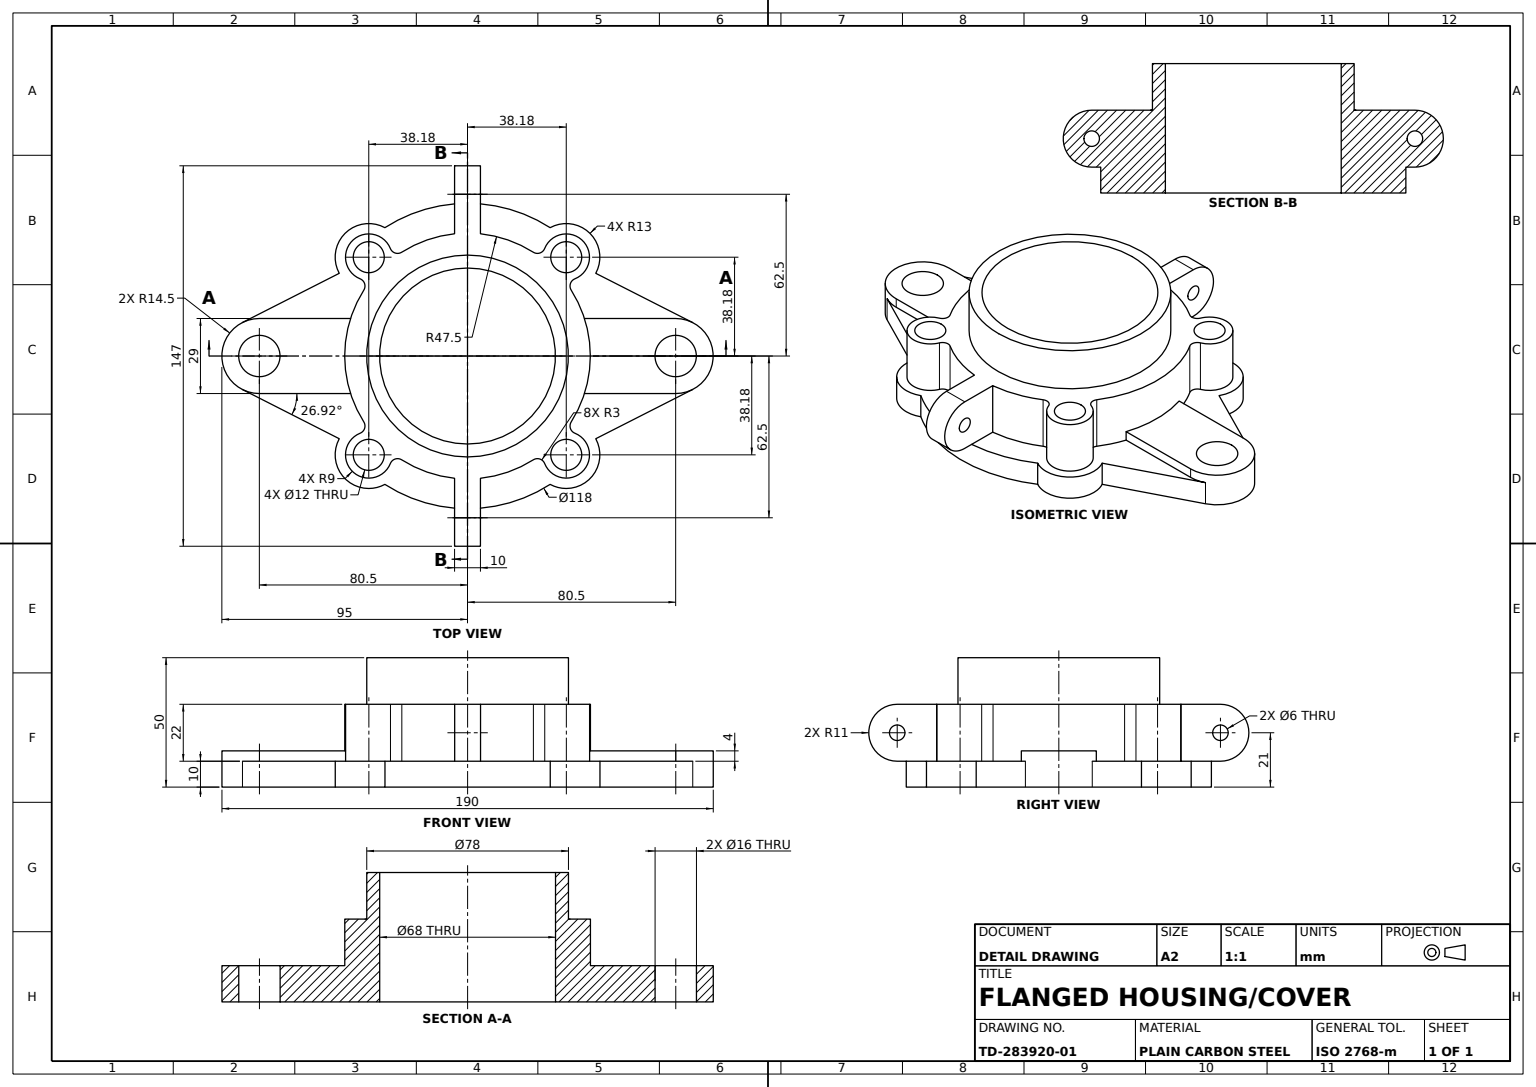
solid
v1 (-80.5,14,14.5)
v2 (-80.5,10,14.5)
e1 v1 v2 LINE
v3 (-45.232732,10,14.5)
e2 v2 v3 LINE
v4 (-45.232732,14,14.5)
e3 v4 v3 LINE
e4 v1 v4 LINE
face PLANE(AX(P(-80.5,14,14.5),D(0,0,-1),D(-1,0,0))) rev [e1 e2 -e3 -e4]
v5 (-38.183766,32,32.183766)
v6 (-38.183766,0,32.183766)
e5 v5 v6 LINE
v7 (-38.183766,0,44.183766)
e6 v6 v7 CIRCLE(AX(P(-38.183766,0,38.183766),D(0,-1,0),D(0,0,1)),6)
v8 (-38.183766,32,44.183766)
e7 v8 v7 LINE
e8 v8 v5 CIRCLE(AX(P(-38.183766,32,38.183766),D(0,1,0),D(0,0,1)),6)
face CYL(AX(P(-38.183766,32,38.183766),D(0,-1,0),D(0,0,-1)),6) rev [e5 e6 -e7 e8]
v9 (-5,10,58.787754)
v10 (5,10,58.787754)
e9 v9 v10 CIRCLE(AX(P(0,10,0),D(0,1,0),D(0,0,1)),59)
v11 (-31.95732,10,49.595662)
e10 v11 v9 CIRCLE(AX(P(0,10,0),D(0,1,0),D(0,0,1)),59)
v12 (-31.95732,0,49.595662)
e11 v11 v12 LINE
v13 (31.95732,0,49.595662)
e12 v12 v13 CIRCLE(AX(P(0,0,0),D(0,1,0),D(0,0,1)),59)
v14 (31.95732,10,49.595662)
e13 v13 v14 LINE
e14 v10 v14 CIRCLE(AX(P(0,10,0),D(0,1,0),D(0,0,1)),59)
face CYL(AX(P(0,10,0),D(0,-1,0),D(0,0,-1)),59) [-e9 -e10 e11 e12 e13 -e14]
v15 (-38.183766,0,51.183766)
v16 (-38.183766,10,51.183766)
e15 v15 v16 LINE
e16 v15 v12 CIRCLE(AX(P(-38.183766,0,38.183766),D(0,1,0),D(0,0,1)),13)
e17 v16 v11 CIRCLE(AX(P(-38.183766,10,38.183766),D(0,1,0),D(0,0,1)),13)
face CYL(AX(P(-38.183766,0,38.183766),D(0,1,0),D(0,0,1)),13) [-e15 e16 -e11 -e17]
v17 (-29.829636,32,41.531678)
v18 (-29.829636,10,41.531678)
e18 v17 v18 LINE
v19 (-27.044926,10,39.647649)
e19 v18 v19 CIRCLE(AX(P(-27.044926,10,42.647649),D(0,-1,0),D(0,0,-1)),3)
v20 (-27.044926,32,39.647649)
e20 v20 v19 LINE
e21 v17 v20 CIRCLE(AX(P(-27.044926,32,42.647649),D(0,-1,0),D(0,0,-1)),3)
face CYL(AX(P(-27.044926,32,42.647649),D(0,-1,0),D(0,0,-1)),3) rev [e18 e19 -e20 -e21]
v21 (38.183766,32,-44.183766)
v22 (38.183766,0,-44.183766)
e22 v21 v22 LINE
v23 (38.183766,0,-32.183766)
e23 v22 v23 CIRCLE(AX(P(38.183766,0,-38.183766),D(0,-1,0),D(0,0,1)),6)
v24 (38.183766,32,-32.183766)
e24 v24 v23 LINE
e25 v24 v21 CIRCLE(AX(P(38.183766,32,-38.183766),D(0,1,0),D(0,0,1)),6)
face CYL(AX(P(38.183766,32,-38.183766),D(0,-1,0),D(0,0,-1)),6) rev [e22 e23 -e24 e25]
v25 (0,50,-39)
v26 (0,32,-39)
e26 v25 v26 LINE
v27 (0,50,39)
e27 v27 v25 CIRCLE(AX(P(0,50,0),D(0,1,0),D(0,0,1)),39)
v28 (0,32,39)
e28 v27 v28 LINE
e29 v28 v26 CIRCLE(AX(P(0,32,0),D(0,1,0),D(0,0,1)),39)
face CYL(AX(P(0,50,0),D(0,-1,0),D(0,0,-1)),39) [-e26 -e27 e28 e29]
v29 (-38.183766,32,-44.183766)
v30 (-38.183766,0,-44.183766)
e30 v29 v30 LINE
v31 (-38.183766,32,-32.183766)
e31 v29 v31 CIRCLE(AX(P(-38.183766,32,-38.183766),D(0,1,0),D(0,0,1)),6)
v32 (-38.183766,0,-32.183766)
e32 v31 v32 LINE
e33 v32 v30 CIRCLE(AX(P(-38.183766,0,-38.183766),D(0,-1,0),D(0,0,1)),6)
face CYL(AX(P(-38.183766,32,-38.183766),D(0,-1,0),D(0,0,-1)),6) rev [-e30 e31 e32 e33]
v33 (29.829636,32,41.531678)
v34 (41.531678,32,29.829636)
e34 v33 v34 CIRCLE(AX(P(38.183766,32,38.183766),D(0,1,0),D(0,0,1)),9)
v35 (29.829636,10,41.531678)
e35 v33 v35 LINE
v36 (41.531678,10,29.829636)
e36 v35 v36 CIRCLE(AX(P(38.183766,10,38.183766),D(0,1,0),D(0,0,1)),9)
e37 v34 v36 LINE
face CYL(AX(P(38.183766,32,38.183766),D(0,-1,0),D(0,0,-1)),9) [-e34 e35 e36 -e37]
v37 (38.183766,0,44.183766)
v38 (38.183766,0,32.183766)
e38 v37 v38 CIRCLE(AX(P(38.183766,0,38.183766),D(0,-1,0),D(0,0,1)),6)
v39 (38.183766,32,32.183766)
e39 v39 v38 LINE
v40 (38.183766,32,44.183766)
e40 v39 v40 CIRCLE(AX(P(38.183766,32,38.183766),D(0,1,0),D(0,0,1)),6)
e41 v40 v37 LINE
face CYL(AX(P(38.183766,32,38.183766),D(0,-1,0),D(0,0,-1)),6) rev [e38 -e39 e40 e41]
e42 v25 v27 CIRCLE(AX(P(0,50,0),D(0,1,0),D(0,0,1)),39)
e43 v26 v28 CIRCLE(AX(P(0,32,0),D(0,1,0),D(0,0,1)),39)
face CYL(AX(P(0,50,0),D(0,-1,0),D(0,0,-1)),39) [-e42 e26 e43 -e28]
v41 (5,10,-62.5)
v42 (-5,10,-62.5)
e44 v41 v42 LINE
v43 (5,10,-58.787754)
e45 v43 v41 LINE
v44 (0,10,-59)
e46 v43 v44 CIRCLE(AX(P(0,10,0),D(0,1,0),D(0,0,1)),59)
v45 (-5,10,-58.787754)
e47 v44 v45 CIRCLE(AX(P(0,10,0),D(0,1,0),D(0,0,1)),59)
e48 v42 v45 LINE
face PLANE(AX(P(0,10,0),D(0,1,0),D(0,0,1))) rev [-e44 -e45 e46 e47 -e48]
v46 (0,50,-34)
v47 (0,50,34)
e49 v46 v47 CIRCLE(AX(P(0,50,0),D(0,1,0),D(0,0,1)),34)
e50 v47 v46 CIRCLE(AX(P(0,50,0),D(0,1,0),D(0,0,1)),34)
face PLANE(AX(P(0,50,0),D(0,1,0),D(0,0,1))) [e42 e27] [-e49 -e50]
v48 (-5,32,-47.236109)
v49 (-5,10,-47.236109)
e51 v48 v49 LINE
v50 (-5,32,-62.5)
e52 v50 v48 LINE
v51 (-5,21,-73.5)
e53 v51 v50 CIRCLE(AX(P(-5,21,-62.5),D(1,0,0),D(0,0,-1)),11)
e54 v42 v51 CIRCLE(AX(P(-5,21,-62.5),D(1,0,0),D(0,0,-1)),11)
e55 v45 v49 LINE
v52 (-5,21,-65.5)
v53 (-5,21,-59.5)
e56 v52 v53 CIRCLE(AX(P(-5,21,-62.5),D(1,0,0),D(0,0,-1)),3)
e57 v53 v52 CIRCLE(AX(P(-5,21,-62.5),D(1,0,0),D(0,0,-1)),3)
face PLANE(AX(P(-5,32,-47.236109),D(1,0,0),D(0,0,-1))) rev [-e51 -e52 -e53 -e54 e48 e55] [e56 e57]
v54 (49.595662,0,-31.95732)
v55 (49.595662,10,-31.95732)
e58 v54 v55 LINE
v56 (87.065615,10,-12.928368)
e59 v56 v55 LINE
v57 (87.065615,0,-12.928368)
e60 v56 v57 LINE
e61 v57 v54 LINE
face PLANE(AX(P(87.065615,10,-12.928368),D(-0.452801048,0,0.891611581),D(0.891611581,0,0.452801048))) rev [e58 -e59 e60 e61]
v58 (-25.438297,32,-40.114125)
v59 (-25.438297,10,-40.114125)
e62 v58 v59 LINE
e63 v48 v58 CIRCLE(AX(P(0,32,0),D(0,1,0),D(0,0,1)),47.5)
e64 v49 v59 CIRCLE(AX(P(0,10,0),D(0,1,0),D(0,0,1)),47.5)
face CYL(AX(P(0,32,0),D(0,-1,0),D(0,0,-1)),47.5) [-e62 -e63 e51 e64]
v60 (5,21,-73.5)
e65 v41 v60 CIRCLE(AX(P(5,21,-62.5),D(1,0,0),D(0,0,-1)),11)
e66 v51 v60 LINE
face CYL(AX(P(-5,21,-62.5),D(1,0,0),D(0,0,-1)),11) [-e65 e44 e54 e66]
v61 (-80.5,14,-8)
v62 (-80.5,14,8)
e67 v61 v62 CIRCLE(AX(P(-80.5,14,0),D(0,1,0),D(0,0,1)),8)
e68 v62 v61 CIRCLE(AX(P(-80.5,14,0),D(0,1,0),D(0,0,1)),8)
v63 (-45.232732,14,-14.5)
v64 (-80.5,14,-14.5)
e69 v63 v64 LINE
e70 v64 v1 CIRCLE(AX(P(-80.5,14,0),D(0,1,0),D(0,0,1)),14.5)
e71 v4 v63 CIRCLE(AX(P(0,14,0),D(0,-1,0),D(0,0,1)),47.5)
face PLANE(AX(P(-80.5,14,0),D(0,1,0),D(0,0,1))) [-e67 -e68] [e69 e70 e4 e71]
v65 (0,0,34)
e72 v47 v65 LINE
v66 (0,0,-34)
e73 v65 v66 CIRCLE(AX(P(0,0,0),D(0,-1,0),D(0,0,1)),34)
e74 v46 v66 LINE
face CYL(AX(P(0,50,0),D(0,-1,0),D(0,0,-1)),34) rev [e72 e73 -e74 e49]
v67 (31.95732,10,-49.595662)
e75 v67 v43 CIRCLE(AX(P(0,10,0),D(0,1,0),D(0,0,1)),59)
v68 (31.95732,0,-49.595662)
e76 v67 v68 LINE
v69 (0,0,-59)
e77 v68 v69 CIRCLE(AX(P(0,0,0),D(0,1,0),D(0,0,1)),59)
e78 v44 v69 LINE
face CYL(AX(P(0,10,0),D(0,-1,0),D(0,0,-1)),59) [-e75 e76 e77 -e78 -e46]
v70 (-38.183766,32,-47.183766)
v71 (-38.183766,10,-47.183766)
e79 v70 v71 LINE
v72 (-29.829636,32,-41.531678)
e80 v72 v70 CIRCLE(AX(P(-38.183766,32,-38.183766),D(0,1,0),D(0,0,1)),9)
v73 (-29.829636,10,-41.531678)
e81 v72 v73 LINE
e82 v73 v71 CIRCLE(AX(P(-38.183766,10,-38.183766),D(0,1,0),D(0,0,1)),9)
face CYL(AX(P(-38.183766,32,-38.183766),D(0,-1,0),D(0,0,-1)),9) [-e79 -e80 e81 e82]
v74 (5,21,-65.5)
e83 v52 v74 LINE
v75 (5,21,-59.5)
e84 v74 v75 CIRCLE(AX(P(5,21,-62.5),D(1,0,0),D(0,0,-1)),3)
e85 v53 v75 LINE
face CYL(AX(P(-5,21,-62.5),D(1,0,0),D(0,0,-1)),3) rev [-e56 e83 e84 -e85]
e86 v7 v6 CIRCLE(AX(P(-38.183766,0,38.183766),D(0,-1,0),D(0,0,1)),6)
e87 v5 v8 CIRCLE(AX(P(-38.183766,32,38.183766),D(0,1,0),D(0,0,1)),6)
face CYL(AX(P(-38.183766,32,38.183766),D(0,-1,0),D(0,0,-1)),6) rev [e7 e86 -e5 e87]
v76 (80.5,14,-8)
v77 (80.5,14,8)
e88 v76 v77 CIRCLE(AX(P(80.5,14,0),D(0,1,0),D(0,0,1)),8)
e89 v77 v76 CIRCLE(AX(P(80.5,14,0),D(0,1,0),D(0,0,1)),8)
v78 (80.5,14,14.5)
v79 (80.5,14,-14.5)
e90 v78 v79 CIRCLE(AX(P(80.5,14,0),D(0,1,0),D(0,0,1)),14.5)
v80 (45.232732,14,-14.5)
e91 v79 v80 LINE
v81 (45.232732,14,14.5)
e92 v80 v81 CIRCLE(AX(P(0,14,0),D(0,-1,0),D(0,0,1)),47.5)
e93 v81 v78 LINE
face PLANE(AX(P(80.5,14,0),D(0,1,0),D(0,0,1))) [-e88 -e89] [e90 e91 e92 e93]
v82 (-45.232732,10,-14.5)
e94 v63 v82 LINE
v83 (-80.5,10,-14.5)
e95 v82 v83 LINE
e96 v64 v83 LINE
face PLANE(AX(P(-80.5,14,-14.5),D(0,0,1),D(1,0,0))) rev [-e69 e94 e95 -e96]
v84 (-80.5,0,8)
e97 v62 v84 LINE
v85 (-80.5,0,-8)
e98 v85 v84 CIRCLE(AX(P(-80.5,0,0),D(0,1,0),D(0,0,1)),8)
e99 v61 v85 LINE
face CYL(AX(P(-80.5,10,0),D(0,-1,0),D(0,0,-1)),8) rev [e97 -e98 -e99 e67]
v86 (-5,32,62.5)
v87 (-5,10,62.5)
e100 v86 v87 CIRCLE(AX(P(-5,21,62.5),D(1,0,0),D(0,0,-1)),11)
v88 (5,10,62.5)
e101 v87 v88 LINE
v89 (5,32,62.5)
e102 v89 v88 CIRCLE(AX(P(5,21,62.5),D(1,0,0),D(0,0,-1)),11)
e103 v86 v89 LINE
face CYL(AX(P(-5,21,62.5),D(1,0,0),D(0,0,-1)),11) [e100 e101 -e102 -e103]
v90 (-31.95732,10,-49.595662)
e104 v45 v90 CIRCLE(AX(P(0,10,0),D(0,1,0),D(0,0,1)),59)
v91 (-31.95732,0,-49.595662)
e105 v69 v91 CIRCLE(AX(P(0,0,0),D(0,1,0),D(0,0,1)),59)
e106 v91 v90 LINE
face CYL(AX(P(0,10,0),D(0,-1,0),D(0,0,-1)),59) [-e104 -e47 e78 e105 e106]
v92 (5,32,47.236109)
v93 (5,10,47.236109)
e107 v92 v93 LINE
v94 (25.438297,10,40.114125)
e108 v93 v94 CIRCLE(AX(P(0,10,0),D(0,1,0),D(0,0,1)),47.5)
v95 (25.438297,32,40.114125)
e109 v95 v94 LINE
e110 v92 v95 CIRCLE(AX(P(0,32,0),D(0,1,0),D(0,0,1)),47.5)
face CYL(AX(P(0,32,0),D(0,-1,0),D(0,0,-1)),47.5) [e107 e108 -e109 -e110]
v96 (-49.595662,10,-31.95732)
v97 (-49.595662,0,-31.95732)
e111 v96 v97 LINE
v98 (-87.065615,0,-12.928368)
e112 v97 v98 LINE
v99 (-87.065615,10,-12.928368)
e113 v99 v98 LINE
e114 v96 v99 LINE
face PLANE(AX(P(-87.065615,10,-12.928368),D(0.452801048,0,0.891611581),D(0.891611581,0,-0.452801048))) rev [e111 e112 -e113 -e114]
e115 v38 v37 CIRCLE(AX(P(38.183766,0,38.183766),D(0,-1,0),D(0,0,1)),6)
e116 v40 v39 CIRCLE(AX(P(38.183766,32,38.183766),D(0,1,0),D(0,0,1)),6)
face CYL(AX(P(38.183766,32,38.183766),D(0,-1,0),D(0,0,-1)),6) rev [e39 e115 -e41 e116]
v100 (40.114125,32,25.438297)
v101 (40.114125,10,25.438297)
e117 v100 v101 LINE
v102 (45.232732,10,14.5)
e118 v101 v102 CIRCLE(AX(P(0,10,0),D(0,1,0),D(0,0,1)),47.5)
e119 v81 v102 LINE
v103 (45.232732,10,-14.5)
e120 v80 v103 LINE
v104 (40.114125,10,-25.438297)
e121 v103 v104 CIRCLE(AX(P(0,10,0),D(0,1,0),D(0,0,1)),47.5)
v105 (40.114125,32,-25.438297)
e122 v105 v104 LINE
e123 v100 v105 CIRCLE(AX(P(0,32,0),D(0,1,0),D(0,0,1)),47.5)
face CYL(AX(P(0,32,0),D(0,-1,0),D(0,0,-1)),47.5) [e117 e118 -e119 -e92 e120 e121 -e122 -e123]
v106 (41.531678,32,-29.829636)
v107 (41.531678,10,-29.829636)
e124 v106 v107 LINE
e125 v105 v106 CIRCLE(AX(P(42.647649,32,-27.044926),D(0,-1,0),D(0,0,-1)),3)
e126 v104 v107 CIRCLE(AX(P(42.647649,10,-27.044926),D(0,-1,0),D(0,0,-1)),3)
face CYL(AX(P(42.647649,32,-27.044926),D(0,-1,0),D(0,0,-1)),3) rev [-e124 -e125 e122 e126]
v108 (-87.065615,10,12.928368)
v109 (-49.595662,10,31.95732)
e127 v108 v109 LINE
e128 v109 v16 CIRCLE(AX(P(-38.183766,10,38.183766),D(0,1,0),D(0,0,1)),13)
v110 (-5,10,47.236109)
e129 v110 v9 LINE
v111 (-25.438297,10,40.114125)
e130 v111 v110 CIRCLE(AX(P(0,10,0),D(0,1,0),D(0,0,1)),47.5)
e131 v19 v111 CIRCLE(AX(P(-27.044926,10,42.647649),D(0,-1,0),D(0,0,-1)),3)
v112 (-41.531678,10,29.829636)
e132 v112 v18 CIRCLE(AX(P(-38.183766,10,38.183766),D(0,1,0),D(0,0,1)),9)
v113 (-40.114125,10,25.438297)
e133 v113 v112 CIRCLE(AX(P(-42.647649,10,27.044926),D(0,-1,0),D(0,0,-1)),3)
e134 v3 v113 CIRCLE(AX(P(0,10,0),D(0,1,0),D(0,0,1)),47.5)
e135 v108 v2 CIRCLE(AX(P(-80.5,10,0),D(0,1,0),D(0,0,1)),14.5)
face PLANE(AX(P(0,10,0),D(0,1,0),D(0,0,1))) [e127 e128 e17 e10 -e129 -e130 -e131 -e19 -e132 -e133 -e134 -e2 -e135]
v114 (-40.114125,32,-25.438297)
v115 (-40.114125,32,25.438297)
e136 v114 v115 CIRCLE(AX(P(0,32,0),D(0,1,0),D(0,0,1)),47.5)
v116 (-40.114125,10,-25.438297)
e137 v114 v116 LINE
e138 v116 v82 CIRCLE(AX(P(0,10,0),D(0,1,0),D(0,0,1)),47.5)
e139 v115 v113 LINE
face CYL(AX(P(0,32,0),D(0,-1,0),D(0,0,-1)),47.5) [-e136 e137 e138 -e94 -e71 e3 e134 -e139]
v117 (27.044926,10,39.647649)
e140 v94 v117 CIRCLE(AX(P(27.044926,10,42.647649),D(0,-1,0),D(0,0,-1)),3)
e141 v10 v93 LINE
v118 (38.183766,10,51.183766)
e142 v14 v118 CIRCLE(AX(P(38.183766,10,38.183766),D(0,1,0),D(0,0,1)),13)
v119 (49.595662,10,31.95732)
e143 v118 v119 CIRCLE(AX(P(38.183766,10,38.183766),D(0,1,0),D(0,0,1)),13)
v120 (87.065615,10,12.928368)
e144 v119 v120 LINE
v121 (80.5,10,14.5)
e145 v121 v120 CIRCLE(AX(P(80.5,10,0),D(0,1,0),D(0,0,1)),14.5)
e146 v102 v121 LINE
e147 v36 v101 CIRCLE(AX(P(42.647649,10,27.044926),D(0,-1,0),D(0,0,-1)),3)
e148 v117 v35 CIRCLE(AX(P(27.044926,10,42.647649),D(0,-1,0),D(0,0,-1)),3)
face PLANE(AX(P(0,10,0),D(0,1,0),D(0,0,1))) [-e140 -e108 -e141 e14 e142 e143 e144 -e145 -e146 -e118 -e147 -e36 -e148]
v122 (-41.531678,10,-29.829636)
e149 v71 v122 CIRCLE(AX(P(-38.183766,10,-38.183766),D(0,1,0),D(0,0,1)),9)
e150 v59 v73 CIRCLE(AX(P(-27.044926,10,-42.647649),D(0,-1,0),D(0,0,-1)),3)
e151 v90 v96 CIRCLE(AX(P(-38.183766,10,-38.183766),D(0,1,0),D(0,0,1)),13)
e152 v83 v99 CIRCLE(AX(P(-80.5,10,0),D(0,1,0),D(0,0,1)),14.5)
e153 v122 v116 CIRCLE(AX(P(-42.647649,10,-27.044926),D(0,-1,0),D(0,0,1)),3)
face PLANE(AX(P(0,10,0),D(0,1,0),D(0,0,1))) [-e149 -e82 -e150 -e64 -e55 e104 e151 e114 -e152 -e95 -e138 -e153]
e154 v9 v87 LINE
v123 (-5,32,47.236109)
e155 v123 v86 LINE
e156 v123 v110 LINE
v124 (-5,21,59.5)
v125 (-5,21,65.5)
e157 v124 v125 CIRCLE(AX(P(-5,21,62.5),D(1,0,0),D(0,0,-1)),3)
e158 v125 v124 CIRCLE(AX(P(-5,21,62.5),D(1,0,0),D(0,0,-1)),3)
face PLANE(AX(P(-5,32,47.236109),D(1,0,0),D(0,0,-1))) rev [e154 -e100 -e155 e156 e129] [e157 e158]
v126 (25.438297,32,-40.114125)
v127 (25.438297,10,-40.114125)
e159 v126 v127 LINE
v128 (5,10,-47.236109)
e160 v127 v128 CIRCLE(AX(P(0,10,0),D(0,1,0),D(0,0,1)),47.5)
v129 (5,32,-47.236109)
e161 v129 v128 LINE
e162 v126 v129 CIRCLE(AX(P(0,32,0),D(0,1,0),D(0,0,1)),47.5)
face CYL(AX(P(0,32,0),D(0,-1,0),D(0,0,-1)),47.5) [e159 e160 -e161 -e162]
e163 v88 v10 LINE
face PLANE(AX(P(0,10,0),D(0,1,0),D(0,0,1))) rev [-e101 -e154 e9 -e163]
v130 (80.5,10,-14.5)
e164 v79 v130 LINE
e165 v130 v103 LINE
face PLANE(AX(P(80.5,14,-14.5),D(0,0,1),D(1,0,0))) rev [-e91 e164 e165 -e120]
v131 (27.044926,32,39.647649)
e166 v131 v117 LINE
e167 v131 v33 CIRCLE(AX(P(27.044926,32,42.647649),D(0,-1,0),D(0,0,-1)),3)
face CYL(AX(P(27.044926,32,42.647649),D(0,-1,0),D(0,0,-1)),3) rev [e166 e148 -e35 -e167]
v132 (-87.065615,0,12.928368)
e168 v98 v132 CIRCLE(AX(P(-80.5,0,0),D(0,1,0),D(0,0,1)),14.5)
e169 v108 v132 LINE
face CYL(AX(P(-80.5,10,0),D(0,-1,0),D(0,0,-1)),14.5) [e152 e113 e168 -e169 e135 -e1 -e70 e96]
e170 v66 v65 CIRCLE(AX(P(0,0,0),D(0,-1,0),D(0,0,1)),34)
face CYL(AX(P(0,50,0),D(0,-1,0),D(0,0,-1)),34) rev [-e72 e50 e74 e170]
e171 v78 v121 LINE
v133 (87.065615,0,12.928368)
e172 v120 v133 LINE
e173 v133 v57 CIRCLE(AX(P(80.5,0,0),D(0,1,0),D(0,0,1)),14.5)
e174 v56 v130 CIRCLE(AX(P(80.5,10,0),D(0,1,0),D(0,0,1)),14.5)
face CYL(AX(P(80.5,10,0),D(0,-1,0),D(0,0,-1)),14.5) [-e164 -e90 e171 e145 e172 e173 -e60 e174]
e175 v34 v100 CIRCLE(AX(P(42.647649,32,27.044926),D(0,-1,0),D(0,0,-1)),3)
face CYL(AX(P(42.647649,32,27.044926),D(0,-1,0),D(0,0,-1)),3) rev [-e117 -e175 e37 e147]
v134 (80.5,0,8)
e176 v77 v134 LINE
v135 (80.5,0,-8)
e177 v76 v135 LINE
e178 v134 v135 CIRCLE(AX(P(80.5,0,0),D(0,1,0),D(0,0,1)),8)
face CYL(AX(P(80.5,10,0),D(0,-1,0),D(0,0,-1)),8) rev [-e176 e89 e177 -e178]
e179 v55 v67 CIRCLE(AX(P(38.183766,10,-38.183766),D(0,1,0),D(0,0,1)),13)
e180 v128 v43 LINE
v136 (29.829636,10,-41.531678)
e181 v136 v127 CIRCLE(AX(P(27.044926,10,-42.647649),D(0,-1,0),D(0,0,-1)),3)
v137 (38.183766,10,-47.183766)
e182 v137 v136 CIRCLE(AX(P(38.183766,10,-38.183766),D(0,1,0),D(0,0,1)),9)
e183 v107 v137 CIRCLE(AX(P(38.183766,10,-38.183766),D(0,1,0),D(0,0,1)),9)
face PLANE(AX(P(0,10,0),D(0,1,0),D(0,0,1))) [e179 e75 -e180 -e160 -e181 -e182 -e183 -e126 -e121 -e165 -e174 e59]
v138 (5,21,65.5)
v139 (5,21,59.5)
e184 v138 v139 CIRCLE(AX(P(5,21,62.5),D(1,0,0),D(0,0,-1)),3)
e185 v139 v138 CIRCLE(AX(P(5,21,62.5),D(1,0,0),D(0,0,-1)),3)
e186 v89 v92 LINE
face PLANE(AX(P(5,32,62.5),D(-1,0,0),D(0,0,1))) rev [-e184 -e185] [e141 -e107 -e186 e102 e163]
e187 v91 v97 CIRCLE(AX(P(-38.183766,0,-38.183766),D(0,1,0),D(0,0,1)),13)
face CYL(AX(P(-38.183766,0,-38.183766),D(0,1,0),D(0,0,1)),13) [e187 -e111 -e151 -e106]
face PLANE(AX(P(80.5,14,14.5),D(0,0,-1),D(-1,0,0))) rev [-e171 -e93 e119 e146]
e188 v31 v29 CIRCLE(AX(P(-38.183766,32,-38.183766),D(0,1,0),D(0,0,1)),6)
e189 v21 v24 CIRCLE(AX(P(38.183766,32,-38.183766),D(0,1,0),D(0,0,1)),6)
v140 (5,32,-62.5)
e190 v140 v50 LINE
e191 v58 v72 CIRCLE(AX(P(-27.044926,32,-42.647649),D(0,-1,0),D(0,0,-1)),3)
v141 (-41.531678,32,-29.829636)
e192 v70 v141 CIRCLE(AX(P(-38.183766,32,-38.183766),D(0,1,0),D(0,0,1)),9)
e193 v141 v114 CIRCLE(AX(P(-42.647649,32,-27.044926),D(0,-1,0),D(0,0,1)),3)
v142 (-41.531678,32,29.829636)
e194 v115 v142 CIRCLE(AX(P(-42.647649,32,27.044926),D(0,-1,0),D(0,0,-1)),3)
e195 v142 v17 CIRCLE(AX(P(-38.183766,32,38.183766),D(0,1,0),D(0,0,1)),9)
v143 (-25.438297,32,40.114125)
e196 v20 v143 CIRCLE(AX(P(-27.044926,32,42.647649),D(0,-1,0),D(0,0,-1)),3)
e197 v143 v123 CIRCLE(AX(P(0,32,0),D(0,1,0),D(0,0,1)),47.5)
e198 v95 v131 CIRCLE(AX(P(27.044926,32,42.647649),D(0,-1,0),D(0,0,-1)),3)
v144 (38.183766,32,-47.183766)
e199 v106 v144 CIRCLE(AX(P(38.183766,32,-38.183766),D(0,1,0),D(0,0,1)),9)
v145 (29.829636,32,-41.531678)
e200 v144 v145 CIRCLE(AX(P(38.183766,32,-38.183766),D(0,1,0),D(0,0,1)),9)
e201 v145 v126 CIRCLE(AX(P(27.044926,32,-42.647649),D(0,-1,0),D(0,0,-1)),3)
e202 v129 v140 LINE
face PLANE(AX(P(-40.415708,32,-32.614346),D(0,1,0),D(0,0,1))) [-e29 -e43] [-e188 -e31] [-e116 -e40] [-e87 -e8] [-e25 -e189] [e190 e52 e63 e191 e80 e192 e193 e136 e194 e195 e21 e196 e197 e155 e103 e186 e110 e198 e167 e34 e175 e123 e125 e199 e200 e201 e162 e202]
e203 v84 v85 CIRCLE(AX(P(-80.5,0,0),D(0,1,0),D(0,0,1)),8)
face CYL(AX(P(-80.5,10,0),D(0,-1,0),D(0,0,-1)),8) rev [e99 -e203 -e97 e68]
e204 v30 v32 CIRCLE(AX(P(-38.183766,0,-38.183766),D(0,-1,0),D(0,0,1)),6)
face CYL(AX(P(-38.183766,32,-38.183766),D(0,-1,0),D(0,0,-1)),6) rev [e30 e204 -e32 e188]
v146 (38.183766,0,51.183766)
e205 v146 v118 LINE
e206 v13 v146 CIRCLE(AX(P(38.183766,0,38.183766),D(0,1,0),D(0,0,1)),13)
face CYL(AX(P(38.183766,0,38.183766),D(0,1,0),D(0,0,1)),13) [e205 -e142 -e13 e206]
face CYL(AX(P(27.044926,32,42.647649),D(0,-1,0),D(0,0,-1)),3) rev [-e198 e109 e140 -e166]
v147 (-49.595662,0,31.95732)
e207 v147 v109 LINE
e208 v147 v15 CIRCLE(AX(P(-38.183766,0,38.183766),D(0,1,0),D(0,0,1)),13)
face CYL(AX(P(-38.183766,0,38.183766),D(0,1,0),D(0,0,1)),13) [-e128 -e207 e208 e15]
e209 v124 v139 LINE
e210 v125 v138 LINE
face CYL(AX(P(-5,21,62.5),D(1,0,0),D(0,0,-1)),3) rev [e209 e185 -e210 -e157]
e211 v145 v136 LINE
face CYL(AX(P(27.044926,32,-42.647649),D(0,-1,0),D(0,0,-1)),3) rev [e181 -e159 -e201 e211]
face CYL(AX(P(-27.044926,32,-42.647649),D(0,-1,0),D(0,0,-1)),3) rev [e150 -e81 -e191 e62]
e212 v142 v112 LINE
face CYL(AX(P(-42.647649,32,27.044926),D(0,-1,0),D(0,0,-1)),3) rev [-e194 e139 e133 -e212]
v148 (49.595662,0,31.95732)
e213 v119 v148 LINE
e214 v148 v133 LINE
face PLANE(AX(P(87.065615,10,12.928368),D(-0.452801048,0,-0.891611581),D(-0.891611581,0,0.452801048))) rev [-e144 e213 e214 -e172]
e215 v23 v22 CIRCLE(AX(P(38.183766,0,-38.183766),D(0,-1,0),D(0,0,1)),6)
face CYL(AX(P(38.183766,32,-38.183766),D(0,-1,0),D(0,0,-1)),6) rev [e189 e24 e215 -e22]
e216 v135 v134 CIRCLE(AX(P(80.5,0,0),D(0,1,0),D(0,0,1)),8)
e217 v132 v147 LINE
e218 v54 v68 CIRCLE(AX(P(38.183766,0,-38.183766),D(0,1,0),D(0,0,1)),13)
e219 v146 v148 CIRCLE(AX(P(38.183766,0,38.183766),D(0,1,0),D(0,0,1)),13)
face PLANE(AX(P(0,0,0),D(0,1,0),D(0,0,1))) rev [-e115 -e38] [-e204 -e33] [-e170 -e73] [-e215 -e23] [e216 e178] [-e208 -e217 -e168 -e112 -e187 -e105 -e77 -e218 -e61 -e173 -e214 -e219 -e206 -e12 -e16] [-e86 -e6] [e203 e98]
e220 v141 v122 LINE
face CYL(AX(P(-38.183766,32,-38.183766),D(0,-1,0),D(0,0,-1)),9) [-e192 e79 e149 -e220]
face PLANE(AX(P(-87.065615,10,12.928368),D(0.452801048,0,-0.891611581),D(-0.891611581,0,-0.452801048))) rev [e207 -e127 e169 e217]
e221 v60 v140 CIRCLE(AX(P(5,21,-62.5),D(1,0,0),D(0,0,-1)),11)
e222 v75 v74 CIRCLE(AX(P(5,21,-62.5),D(1,0,0),D(0,0,-1)),3)
face PLANE(AX(P(5,32,-62.5),D(-1,0,0),D(0,0,1))) rev [e221 -e202 e161 e180 e45 e65] [-e222 -e84]
face CYL(AX(P(-5,21,-62.5),D(1,0,0),D(0,0,-1)),3) rev [-e83 -e57 e85 e222]
e223 v143 v111 LINE
face CYL(AX(P(-27.044926,32,42.647649),D(0,-1,0),D(0,0,-1)),3) rev [-e196 e20 e131 -e223]
e224 v144 v137 LINE
face CYL(AX(P(38.183766,32,-38.183766),D(0,-1,0),D(0,0,-1)),9) [-e200 e224 e182 -e211]
face CYL(AX(P(38.183766,32,-38.183766),D(0,-1,0),D(0,0,-1)),9) [-e199 e124 e183 -e224]
face CYL(AX(P(80.5,10,0),D(0,-1,0),D(0,0,-1)),8) rev [-e216 -e177 e88 e176]
face CYL(AX(P(38.183766,0,-38.183766),D(0,1,0),D(0,0,1)),13) [-e76 -e179 -e58 e218]
face CYL(AX(P(-5,21,-62.5),D(1,0,0),D(0,0,-1)),11) [e53 -e190 -e221 -e66]
face CYL(AX(P(0,32,0),D(0,-1,0),D(0,0,-1)),47.5) [e223 e130 -e156 -e197]
face CYL(AX(P(-38.183766,32,38.183766),D(0,-1,0),D(0,0,-1)),9) [e132 -e18 -e195 e212]
face CYL(AX(P(-42.647649,32,-27.044926),D(0,-1,0),D(0,0,-1)),3) rev [e153 -e137 -e193 e220]
face CYL(AX(P(38.183766,0,38.183766),D(0,1,0),D(0,0,1)),13) [-e205 e219 -e213 -e143]
face CYL(AX(P(-5,21,62.5),D(1,0,0),D(0,0,-1)),3) rev [e184 -e209 -e158 e210]
